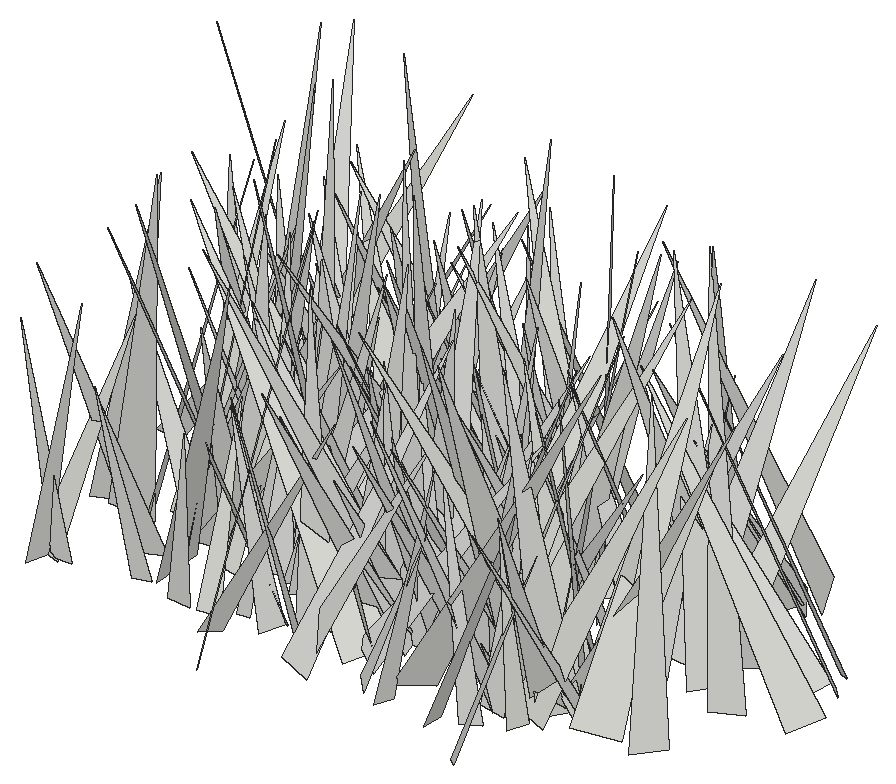
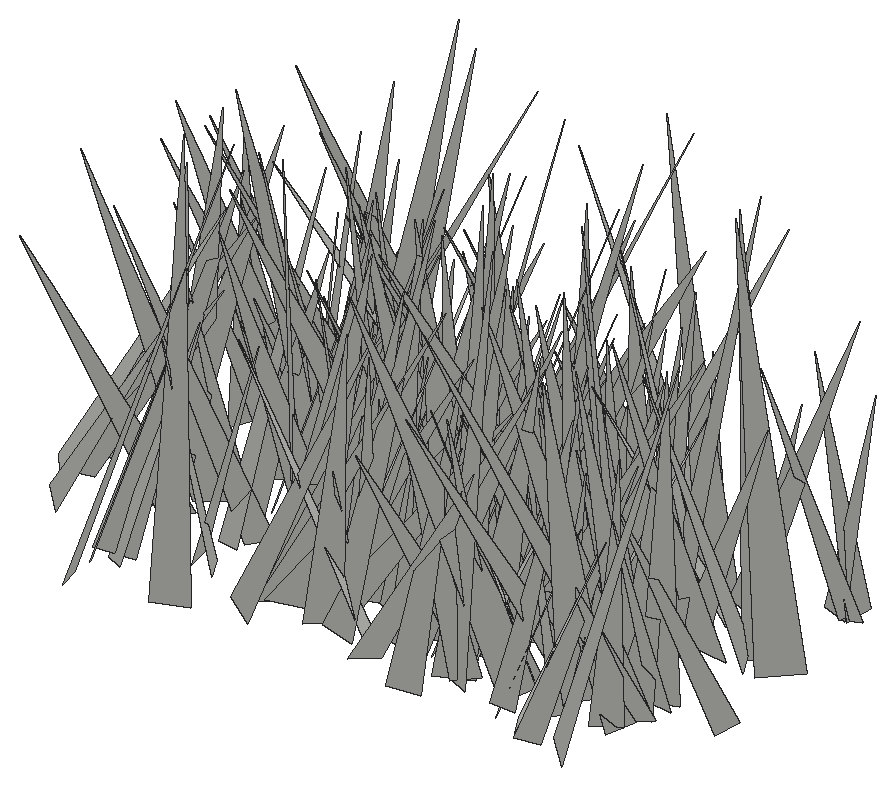
# SketchUp Ruby script. Lengths in inches.
U = 1.inch
M = Sketchup.active_model
def pt(a) = Geom::Point3d.new(a.map { |v| v * U })
def face(e, loops, mat)
  f = e.add_face(loops[0].map { |a| pt(a) })
  loops[1..].each { |l| e.add_face(l.map { |a| pt(a) }).erase! }
  f.material = f.back_material = mat if mat
  f
end
# faces: each face lists its corners as indices into pts; further lists are holes
def faces(e, pts, list, mat = nil) = list.each { |f| face(e, (f[0].is_a?(Array) ? f : [f]).map { |l| l.map { |i| pts[i] } }, mat) }
# xy, xz, yz: faces in a plane at the given z, y or x. An outline is a flat list of corners, or four numbers for a rectangle; further outlines are holes
def ring(l) = l.size == 4 ? [[l[0], l[1]], [l[2], l[1]], [l[2], l[3]], [l[0], l[3]]] : l.each_slice(2).to_a
def flat(e, list, mat, &to3) = list.each { |f| face(e, (f[0].is_a?(Array) ? f : [f]).map { |l| ring(l).map { |u, v| to3.(u, v) } }, mat) }
def xy(e, z, list, mat = nil) = flat(e, list, mat) { |x, y| [x, y, z] }
def xz(e, y, list, mat = nil) = flat(e, list, mat) { |x, z| [x, y, z] }
def yz(e, x, list, mat = nil) = flat(e, list, mat) { |y, z| [x, y, z] }
def lines(e, pts, list) = list.each { |a, b| e.add_line(pt(pts[a]), pt(pts[b])) }
# prism: a flat outline (further loops are holes) pulled along v
def prism(e, loops, v, mat = nil)
  f = face(e, loops, mat); d = Geom::Vector3d.new(v.map { |x| x * U })
  f.pushpull(f.normal.samedirection?(d) ? d.length : -d.length)
end
def box(e, o, s, mat = nil) = prism(e, [[o, [o[0] + s[0], o[1], o[2]], [o[0] + s[0], o[1] + s[1], o[2]], [o[0], o[1] + s[1], o[2]]]], [0, 0, s[2]], mat)
def at(x, y, z, deg = 0) = Geom::Transformation.translation(pt([x, y, z])) * Geom::Transformation.rotation(ORIGIN, Z_AXIS, deg.degrees)
def axes(o, x, y, z) = Geom::Transformation.new([*x, 0, *y, 0, *z, 0, *pt(o).to_a, 1])
def part(name) = M.definitions.add(name)
# library, detail: a bought-in or finely detailed component or shape, given as its bounding box
def library(name, o, s) = part(name).tap { |d| box(d.entities, o, s) }
def detail(e, o, s) = box(e.add_group.entities, o, s)
def put(e, d, t, mat = nil) = e.add_instance(d, t).tap { |i| i.material = mat if mat }
def group(e, t, mat = nil) = e.add_group.tap { |g| g.transformation = t; g.material = mat if mat }.entities
root = M.entities
c1 = part("fur_instance\#9")
p = [[0.8125,0,1.79],[0.67,-0.02,1.48],[0,-0.11,0],[0,0.11,0]]
faces(c1.entities,p,[[0,1,2,3]])
put(root,c1,axes([508.12,72.6,-21.86],[0.58274,-3.68979,0.92218],[-3.78198,-0.46356,0.53511],[0.40205,0.98748,3.697]))
put(root,c1,axes([511.35,69.62,-21.66],[6.37842,4.90538,1.53696],[4.59516,-6.53882,1.79932],[-2.30422,0.53885,7.84279]))
put(root,c1,axes([516.26,72.1,-21.86],[2.61371,2.45973,0.53308],[2.49517,-2.43181,-1.01309],[0.32949,-1.09634,3.44317]))
put(root,c1,axes([512.71,73.15,-21.86],[-3.88391,-3.01754,1.00768],[-2.99103,4.00531,0.46572],[1.08383,0.24005,4.89626]))
put(root,c1,axes([506.625,74.36,-21.86],[8.18505,-1.50624,0.16494],[-1.43272,-7.98824,-1.85106],[-0.49323,-1.79175,8.11402]))
put(root,c1,axes([517.57,71.6,-21.86],[4.20313,-0.16718,1.34956],[-0.39887,-4.34286,0.70427],[-1.30006,0.79192,4.14708]))
put(root,c1,axes([503.32,72.43,-21.86],[-0.94166,-4.10224,1.61468],[-4.38512,0.70145,-0.77524],[-0.45421,1.73259,4.13692]))
put(root,c1,axes([502.62,72.03,-21.86],[4.80103,-0.44543,1.50068],[-0.59366,-4.99749,0.41591],[-1.44845,0.57184,4.80368]))
put(root,c1,axes([520.4375,73.95,-21.86],[-5.1626,-2.88411,0.4563],[-2.82641,5.16852,0.6903],[0.7333,-0.3834,5.87316]))
put(root,c1,axes([513.81,71.89,-21.66],[2.98745,4.37857,0.43851],[4.21633,-2.69647,-1.80015],[1.25963,-1.35874,4.98559]))
put(root,c1,axes([522.24,74.51,-21.86],[2.51881,-4.55482,0.15905],[-4.51842,-2.51942,-0.59372],[-0.59628,-0.14918,5.17091]))
put(root,c1,axes([510.13,71.75,-21.86],[4.70172,-1.10111,0.26171],[-1.12934,-4.49092,1.39405],[0.07438,1.41645,4.62334]))
put(root,c1,axes([506.19,73.04,-21.86],[-0.09942,-3.58739,1.13729],[-3.70553,-0.10534,-0.65623],[-0.65715,1.13676,3.52826]))
put(root,c1,axes([523.46,74.95,-21.86],[-3.70308,-3.24105,0.05421],[-3.08159,3.54543,1.46762],[1.00557,-1.07036,4.69716]))
put(root,c1,axes([520.76,72.2,-21.86],[-0.54656,4.2534,1.19948],[4.32093,0.26075,1.04426],[-0.92722,-1.29209,4.15928]))
put(root,c1,axes([515.43,75,-21.66],[1.43774,-5.64122,0.58152],[-5.34924,-1.54822,-1.79367],[-1.88339,0.09091,5.53834]))
put(root,c1,axes([522.07,73.05,-21.86],[-3.10303,1.40825,1.48641],[1.65077,3.31728,0.3033],[1.21143,-0.91317,3.39411]))
put(root,c1,axes([511.62,73.125,-21.86],[-3.58724,1.8714,1.40372],[2.1412,3.66165,0.59026],[0.94225,-1.19623,4.00275]))
put(root,c1,axes([520.34,76.11,-21.86],[6.29678,-5.28708,1.00032],[-4.88133,-6.26054,-2.36253],[-2.26416,-1.20654,7.87535]))
put(root,c1,axes([511.5,73.86,-21.86],[-4.9129,-5.75828,0.52895],[-5.68371,4.68095,-1.83254],[-1.06438,1.58274,7.34412]))
put(root,c1,axes([515.98,75.3,-21.66],[-8.04638,-2.10125,0.20494],[-2.02323,7.90531,1.61682],[0.60315,-1.51404,8.15753]))
put(root,c1,axes([517.01,75.45,-21.66],[-6.19203,-3.31038,1.54754],[-2.85802,6.28451,2.00782],[2.2771,-1.114,6.72819]))
put(root,c1,axes([505.65,74.35,-21.66],[-0.4063,-5.76079,1.26429],[-5.69006,0.04941,-1.60344],[-1.5519,1.32705,5.54804]))
put(root,c1,axes([502.58,72.48,-21.86],[0.61438,4.77457,1.24038],[4.786,-0.27399,-1.3159],[1.1955,-1.35681,4.63059]))
put(root,c1,axes([523.04,75.625,-21.86],[-8.10416,-1.22815,0.06312],[-1.16757,7.81624,2.17553],[0.38615,-2.14192,7.90272]))
put(root,c1,axes([519.85,71.31,-21.66],[6.47636,2.00005,0.90058],[1.74291,-6.39683,1.67254],[-1.33173,1.35459,6.56857]))
put(root,c1,axes([517.88,72.83,-21.66],[7.15691,-3.14413,0.26361],[-3.09126,-6.8566,2.14652],[0.63178,2.06831,7.5166]))
put(root,c1,axes([519.76,76.26,-21.86],[0.59961,-8.00132,0.48644],[-8.01433,-0.60861,-0.13198],[-0.1682,0.47514,8.02267]))
put(root,c1,axes([518.91,75.29,-21.86],[0.11807,-5.18176,0.38422],[-4.95689,-0.22756,-1.54584],[-1.55804,0.33133,4.94722]))
put(root,c1,axes([509.3,72.66,-21.86],[-0.85461,3.70026,0.75554],[3.7566,0.91253,-0.21994],[0.38824,-0.68446,3.79129]))
put(root,c1,axes([522.61,74.59,-21.86],[4.49335,-4.83843,2.48866],[-4.8443,-5.0271,-1.02712],[-2.47721,1.05444,6.5227]))
put(root,c1,axes([513.84,71.52,-21.86],[1.69788,6.23349,0.03172],[6.16311,-1.67374,-0.97718],[0.93461,-0.28707,6.38626]))
put(root,c1,axes([520.75,73.36,-21.86],[0.78552,4.64999,1.51438],[4.88897,-0.70993,-0.35606],[0.11721,-1.55126,4.70241]))
put(root,c1,axes([519.375,76.59,-21.86],[-4.17954,-4.03403,0.06779],[-3.83281,4.00041,1.74723],[1.26,-1.21235,5.53978]))
put(root,c1,axes([521.85,69.87,-21.86],[5.70548,5.18554,0.14342],[4.71826,-5.27598,3.06024],[-2.15603,2.1765,7.07653]))
put(root,c1,axes([512.72,74.08,-21.86],[-1.61639,5.70202,2.80279],[6.31476,1.76115,0.05886],[0.70173,-2.71416,5.92641]))
put(root,c1,axes([515.04,76.29,-21.66],[3.98276,-1.20965,1.22676],[-0.42908,-3.68899,-2.24451],[-1.66855,-1.93873,3.5054]))
put(root,c1,axes([514.28,75.85,-21.86],[-4.07436,-2.22938,0.28557],[-2.14023,4.02883,0.91657],[0.68639,-0.67121,4.55307]))
put(root,c1,axes([514.71,74.17,-21.66],[-5.12266,-6.1706,2.10185],[-6.50165,4.64284,-2.21548],[-0.47189,3.01719,7.70776]))
put(root,c1,axes([515.17,73.78,-21.86],[-5.23637,6.32875,0.17784],[5.87309,4.76933,3.20385],[-2.36465,-2.16904,7.5636]))
put(root,c1,axes([515.23,73.57,-21.86],[2.725,5.40327,0.30402],[4.86473,-2.29653,-2.78814],[2.3711,-1.498,5.37096]))
put(root,c1,axes([518.57,75.48,-21.86],[-1.2496,-4.95098,2.04852],[-4.91628,1.89585,1.58307],[2.13046,1.47094,4.85465]))
put(root,c1,axes([507.4,76.77,-21.86],[4.3108,-3.69492,0.61953],[-3.55093,-4.33068,-1.12044],[-1.19463,-0.46051,5.56597]))
put(root,c1,axes([521.83,73.84,-21.86],[0.86928,6.52033,1.58307],[6.24969,-0.2059,-2.58369],[2.44176,-1.79425,6.04937]))
put(root,c1,axes([503.125,76.37,-21.86],[1.84601,-7.44066,1.73932],[-7.59322,-1.58595,1.27441],[0.85535,1.97933,7.55956]))
put(root,c1,axes([515.2,76.85,-21.86],[2.62732,-3.98087,0.28129],[-3.95197,-2.64215,-0.47983],[-0.55532,-0.03119,4.74551]))
put(root,c1,axes([510.52,72.98,-21.66],[2.07794,4.44656,0.23399],[4.16362,-2.03187,1.63715],[-1.57826,0.49406,4.62704]))
put(root,c1,axes([526.51,74.42,-21.86],[-5.32179,3.05618,1.70346],[3.04909,5.5718,-0.47069],[1.71611,-0.42222,6.11884]))
put(root,c1,axes([502.13,76.76,-21.86],[4.60789,-6.31495,1.14074],[-6.41656,-4.51508,0.92427],[0.08686,1.46561,7.76253]))
put(root,c1,axes([505.51,78.7,-21.86],[-3.16063,-7.46069,0.64697],[-7.21635,3.22195,1.90087],[2.00118,-0.16476,7.87643]))
put(root,c1,axes([515.02,75.65,-21.86],[-0.34045,4.62028,2.07312],[5.05885,0.21591,0.34957],[-0.23002,-2.08976,4.6196]))
put(root,c1,axes([516.96,74.91,-21.86],[3.82826,-1.89723,1.31218],[-2.241,-3.66166,1.2438],[-0.54703,1.72325,4.08754]))
put(root,c1,axes([505.73,76.51,-21.86],[3.31192,-3.28223,0.0309],[-3.2384,-3.26025,0.79144],[0.53549,0.5836,4.59516]))
put(root,c1,axes([513.31,76.02,-21.86],[5.02607,-4.57327,2.19343],[-4.92834,-5.13329,0.59007],[-1.19892,1.92923,6.76964]))
put(root,c1,axes([523.01,75.75,-21.86],[1.98838,-4.24744,1.75797],[-4.57109,-1.62434,1.24561],[0.4862,2.09896,4.52138]))
put(root,c1,axes([520.94,78.43,-21.86],[-3.46675,-5.54657,1.13696],[-5.08588,3.63649,2.23277],[2.48816,-0.29493,6.14797]))
put(root,c1,axes([522.9,75.58,-21.86],[-4.62696,-2.40171,1.71965],[-2.7299,4.69747,-0.78458],[1.12828,1.51649,5.15378]))
put(root,c1,axes([514.03,76.47,-21.86],[-4.61226,3.61546,0.79034],[3.61757,4.1381,2.18138],[-0.78062,-2.18488,5.43931]))
put(root,c1,axes([519,74.41,-21.86],[-5.68198,1.58826,2.45655],[1.00817,6.10119,-1.61279],[2.74605,1.04639,5.67506]))
put(root,c1,axes([519.86,79.15,-21.86],[-5.63617,-2.55407,1.20627],[-1.85262,5.37498,2.72438],[2.13217,-2.08115,5.55585]))
put(root,c1,axes([522.65,75.18,-21.86],[6.21247,-1.9108,0.54363],[-1.98453,-5.88708,1.9863],[0.09123,2.05733,6.18874]))
put(root,c1,axes([506.47,76.24,-21.86],[3.95823,-3.37287,0.12226],[-3.1364,-3.60629,2.0534],[1.24667,1.63622,4.7778]))
put(root,c1,axes([517.1875,77.24,-21.66],[-2.08811,-4.65792,0.59921],[-4.45757,1.75934,-1.85749],[-1.47829,1.27435,4.7546]))
put(root,c1,axes([521.63,76.63,-21.86],[-4.54367,3.48057,1.82928],[3.81076,4.58683,0.73803],[0.96889,-1.71821,5.67579]))
put(root,c1,axes([506.05,76.54,-21.86],[-3.48001,3.233,0.8636],[3.33945,3.27515,1.19585],[-0.21495,-1.45934,4.59703]))
put(root,c1,axes([516.31,74.93,-21.66],[1.43872,7.93621,2.15807],[7.82752,-1.99366,2.11323],[-2.52399,-1.65906,7.7838]))
put(root,c1,axes([509.97,76.45,-21.86],[2.74788,4.31889,0.7575],[4.17328,-2.30167,-2.01583],[1.34551,-1.68135,4.70533]))
put(root,c1,axes([508.06,75.3,-21.86],[0.74131,3.87524,0.12897],[3.87698,-0.74271,0.03187],[-0.05555,-0.12068,3.94537]))
put(root,c1,axes([507.4375,77.28,-21.86],[-4.12278,4.06528,3.37823],[4.64279,4.83304,-0.14992],[2.52655,-2.24755,5.78803]))
put(root,c1,axes([512.39,78.32,-21.86],[-0.32554,-5.06602,0.7464],[-4.99056,0.14633,-1.18345],[-1.14716,0.80105,4.9366]))
put(root,c1,axes([524.4,74.24,-21.86],[-3.86216,7.0455,1.20437],[6.7899,4.04407,-1.88376],[2.2331,-0.11104,7.81068]))
put(root,c1,axes([515.91,76.46,-21.86],[-0.78367,4.54033,1.31363],[4.69244,0.5877,0.76808],[-0.56674,-1.41222,4.54299]))
put(root,c1,axes([506.01,75.78,-21.86],[6.26441,4.08516,1.86388],[4.05019,-6.52197,0.68206],[-1.9387,-0.42509,7.44756]))
put(root,c1,axes([509.68,77.84,-21.86],[-4.95355,2.49117,1.9463],[2.93301,4.97148,1.10159],[1.17959,-1.90003,5.43416]))
put(root,c1,axes([522.27,78.33,-21.86],[-3.91317,-2.34388,0.53173],[-2.28614,3.94348,0.55853],[0.74167,-0.21123,4.52711]))
put(root,c1,axes([518.65,75.03,-21.66],[2.72489,7.5123,0.23605],[7.26372,-2.56761,-2.13568],[1.931,-0.94238,7.70056]))
put(root,c1,axes([509.48,76.12,-21.86],[-0.20928,5.81187,1.2771],[5.90875,0.05179,0.73257],[-0.70395,-1.2931,5.76932]))
put(root,c1,axes([510.41,76.12,-21.86],[5.34451,-1.51745,2.02584],[-2.07356,-5.33917,1.4711],[-1.45157,2.03988,5.35746]))
put(root,c1,axes([523.12,76.59,-21.86],[0.51844,5.23573,1.343],[5.13497,-0.0558,-1.76472],[1.68777,-1.43851,4.95655]))
put(root,c1,axes([512.31,78.95,-21.86],[0.02895,-4.95019,0.58964],[-4.94989,0.0415,0.59139],[0.59214,0.58889,4.91483]))
put(root,c1,axes([518.45,76.64,-21.86],[-4.21104,-1.2398,0.43934],[-1.31531,3.95873,-1.43574],[-0.00925,1.50143,4.14832]))
put(root,c1,axes([517.09,77.91,-21.86],[3.85978,2.30102,0.3483],[2.28006,-3.60384,-1.45862],[0.46617,-1.42533,4.2503]))
put(root,c1,axes([509.1,77.8,-21.86],[-4.69197,-2.31538,0.05263],[-2.28134,4.60011,-1.00642],[-0.39908,0.92541,5.13447]))
put(root,c1,axes([506.0625,74.81,-21.66],[4.52328,4.39752,0.22155],[4.10164,-4.32376,2.0806],[-1.60118,1.34692,5.95561]))
put(root,c1,axes([513.91,78.67,-21.86],[3.13383,-5.16211,1.39491],[-5.34355,-3.08346,0.59403],[-0.19921,1.50298,6.00961]))
put(root,c1,axes([510.9375,75.66,-21.86],[-6.51752,1.2418,2.00991],[0.54856,6.53189,-2.25684],[2.29801,1.9627,6.23913]))
put(root,c1,axes([511.25,78.33,-21.86],[-3.24563,2.42896,0.17461],[2.25293,2.88449,1.75171],[-0.92447,-1.49811,3.65588]))
put(root,c1,axes([514.92,80.65,-21.86],[-0.43608,-7.58063,0.50958],[-7.59761,0.43802,0.01424],[0.04352,0.50791,7.59315]))
put(root,c1,axes([510.28,77.16,-21.86],[-3.93894,0.78438,0.2139],[0.7314,3.88076,-0.76228],[0.35506,0.70765,3.94328]))
put(root,c1,axes([515.53,78.02,-21.86],[-4.0044,1.49429,0.5536],[1.5481,4.00291,0.3933],[0.37782,-0.56428,4.25599]))
put(root,c1,axes([514.53,78.76,-21.86],[-1.30736,-3.53096,1.01989],[-3.67333,1.2908,-0.2398],[0.12042,1.04076,3.75757]))
put(root,c1,axes([513.12,80.63,-21.86],[-3.83453,-4.44323,0.31037],[-4.29048,3.7947,1.3169],[1.19597,-0.63261,5.71941]))
put(root,c1,axes([518.69,78.18,-21.86],[3.7348,-2.45498,0.02516],[-2.33086,-3.53122,1.44009],[0.77113,1.21649,4.23106]))
put(root,c1,axes([509.13,77.04,-21.86],[2.12896,3.50938,0.78952],[3.35263,-2.26833,1.04217],[-1.30344,-0.10245,3.97015]))
put(root,c1,axes([520.75,76.76,-21.66],[6.22186,3.72093,2.03459],[3.43335,-6.54009,1.46143],[-2.48938,0.27987,7.10078]))
put(root,c1,axes([519.51,78.05,-21.86],[7.2049,-3.47591,1.96261],[-3.83046,-7.15988,1.38131],[-1.1231,2.12096,7.87937]))
put(root,c1,axes([511.93,82.83,-21.86],[-6.50454,-4.83681,0.42708],[-4.2184,5.98256,3.50717],[2.40464,-2.5885,7.30777]))
put(root,c1,axes([503.68,76.625,-21.86],[5.51365,3.20537,1.24598],[2.89904,-5.59864,1.57419],[-1.84998,0.77981,6.18035]))
put(root,c1,axes([521.63,81.5625,-21.66],[-2.90473,-5.90083,0.221],[-5.68544,2.86131,1.67173],[1.5951,-0.54696,6.36102]))
put(root,c1,axes([514.91,77.8,-21.66],[2.90433,5.023,0.38727],[4.82562,-2.64532,-1.87916],[1.44702,-1.25991,5.48948]))
put(root,c1,axes([522.5625,79.43,-21.86],[-4.35819,2.96505,1.59627],[3.3258,4.19926,1.28011],[0.52792,-1.97688,5.11338]))
put(root,c1,axes([525.29,80.72,-21.86],[1.43067,-7.01564,1.7352],[-6.90944,-1.84641,-1.76845],[-2.11892,1.28394,6.9382]))
put(root,c1,axes([529.43,79.04,-21.86],[-4.14935,5.21761,0.66717],[4.85978,3.47746,3.02911],[-2.01273,-2.35998,5.93844]))
put(root,c1,axes([512.66,82.05,-21.86],[5.40488,-4.57462,0.50738],[-4.27322,-5.27816,-2.06831],[-1.71004,-1.26929,6.77215]))
put(root,c1,axes([514.7,77.93,-21.86],[-3.77046,5.93467,2.17976],[6.06315,4.1134,-0.71146],[1.79161,-1.43096,6.99504]))
put(root,c1,axes([518.43,79.07,-21.86],[0.00091,-3.67707,1.93886],[-4.08733,0.35251,0.67045],[0.75747,1.90654,3.61543]))
put(root,c1,axes([504.85,77.16,-21.86],[0.72086,7.11073,0.81641],[7.15729,-0.71063,-0.13028],[0.04812,-0.82534,7.14599]))
put(root,c1,axes([508.7,78.96,-21.66],[-2.86629,5.19134,1.30889],[5.27356,2.48156,1.70596],[-0.92348,-1.94182,5.67938]))
put(root,c1,axes([509.05,77.47,-21.66],[-0.59602,7.49567,1.64856],[6.68012,1.32078,-3.59019],[3.77872,-1.15261,6.60687]))
put(root,c1,axes([525.4375,79.125,-21.86],[-5.88987,4.84378,2.23578],[5.14185,6.04195,0.45575],[1.42207,-1.78441,7.61217]))
put(root,c1,axes([523.4,78.66,-21.86],[0.22863,4.55848,1.01522],[4.65358,-0.13679,-0.43379],[0.39321,-1.03161,4.54355]))
put(root,c1,axes([504.91,80.97,-21.66],[1.45023,-6.39796,1.08768],[-6.25164,-1.07813,1.99368],[1.74182,1.45734,6.24998]))
put(root,c1,axes([504.21,82.1,-21.86],[2.77965,-6.05851,0.20454],[-6.05263,-2.78627,-0.276],[-0.3362,0.0706,6.66001]))
put(root,c1,axes([510.05,80.24,-21.86],[-6.653,2.83628,0.09553],[2.75112,6.38619,1.99099],[-0.69638,-1.86767,6.95291]))
put(root,c1,axes([512.22,80.92,-21.86],[-0.4517,-7.27096,2.0225],[-7.50286,0.65147,0.6664],[0.81515,1.96726,7.25444]))
put(root,c1,axes([508.56,79.94,-21.86],[6.38697,-1.69717,1.73981],[-1.81592,-6.58358,0.24416],[-1.61547,0.69051,6.6041]))
put(root,c1,axes([517.57,76.93,-21.86],[-1.37451,8.097,0.63904],[7.82187,1.49419,-2.10823],[2.18815,-0.25501,7.93763]))
put(root,c1,axes([518.75,78.4375,-21.86],[3.29752,4.92899,1.52703],[4.76096,-3.60504,1.35547],[-1.98997,-0.45731,5.77332]))
put(root,c1,axes([505.89,80.25,-21.86],[4.80804,6.17674,2.98381],[6.78482,-4.81897,-0.95722],[-1.01068,-2.96612,7.76873]))
put(root,c1,axes([526.88,78.07,-21.86],[-0.02832,7.80203,1.3013],[7.5934,-0.33756,2.1891],[-2.2148,-1.25708,7.48868]))
put(root,c1,axes([509.68,78.04,-21.86],[-7.86516,0.65945,1.92725],[0.13584,7.83978,-2.12819],[2.03241,2.02799,7.60042]))
put(root,c1,axes([508.59,80.11,-21.86],[3.89931,-1.45547,0.98195],[-1.58431,-3.9476,0.44006],[-0.75669,0.76505,4.13877]))
put(root,c1,axes([528.46,80.85,-21.66],[-4.24155,2.82864,0.08548],[2.61337,3.85608,2.07369],[-1.08573,-1.76881,4.65744]))
put(root,c1,axes([504.07,80.75,-21.86],[2.29625,-5.32789,2.30917],[-5.72704,-2.48806,-0.04565],[-0.95905,2.10109,5.80148]))
put(root,c1,axes([515.39,81.09,-21.86],[3.99451,-5.40043,2.70776],[-5.64329,-4.49426,-0.63847],[-2.15638,1.75774,6.68679]))
put(root,c1,axes([515.27,81.3,-21.86],[-1.72033,-4.15588,1.09836],[-4.2769,1.77348,0.01157],[0.4311,1.01028,4.49785]))
put(root,c1,axes([508.74,79.99,-21.86],[0.17252,3.92598,1.26935],[3.97591,-0.49782,0.99933],[-1.10305,-1.18034,3.80058]))
put(root,c1,axes([517.62,81.25,-21.86],[-2.41735,-5.08882,0.8159],[-4.81582,1.90935,-2.35956],[-1.83565,1.69223,5.11586]))
put(root,c1,axes([509.97,81.28,-21.86],[-5.02237,2.51021,1.68016],[2.86774,4.98644,1.12241],[0.94877,-1.78398,5.50142]))
put(root,c1,axes([504.375,81.58,-21.66],[1.31964,-4.20384,0.49444],[-3.9297,-1.02429,1.77946],[1.57296,0.96785,4.03079]))
put(root,c1,axes([501.02,80.96,-21.66],[2.58418,-3.37784,0.00054],[-2.92311,-2.23595,2.1316],[1.69269,1.29557,3.68023]))
put(root,c1,axes([518,79.82,-21.86],[-6.07575,2.79462,0.62219],[2.80321,6.10345,-0.04049],[0.58225,-0.22305,6.68752]))
put(root,c1,axes([529.08,81.14,-21.66],[-5.24888,-4.54366,0.15791],[-4.36596,4.97023,-2.11085],[-1.26815,1.69482,6.61361]))
put(root,c1,axes([515.91,79.99,-21.86],[3.41828,7.22194,2.57308],[7.56489,-3.63472,0.1519],[-1.24484,-2.25703,7.98861]))
put(root,c1,axes([507.99,80.13,-21.86],[-2.49427,4.27012,1.59064],[4.35584,2.76683,-0.59729],[1.33819,-1.04698,4.90903]))
put(root,c1,axes([510.9,79.18,-21.86],[-2.09774,5.99421,0.07606],[5.73274,1.98235,1.88224],[-1.75272,-0.69034,6.06533]))
put(root,c1,axes([508.17,79.82,-21.86],[4.9565,-0.0282,0.53243],[-0.1703,-4.80111,1.33099],[-0.50525,1.34155,4.77453]))
put(root,c1,axes([516.57,82.39,-21.86],[-3.87512,-3.17972,0.32504],[-3.163,3.88842,0.32938],[0.4601,-0.04943,5.00187]))
put(root,c1,axes([524.2,84.34,-21.66],[4.00993,-5.51552,0.33203],[-5.14979,-3.87921,-2.24547],[-2.00271,-1.06842,6.43882]))
put(root,c1,axes([513.36,82.78,-21.86],[-2.38013,-2.88459,0.25848],[-2.75196,2.35686,0.96161],[0.90246,-0.42079,3.61403]))
put(root,c1,axes([523.85,79.53,-21.66],[-1.22058,7.14872,1.6543],[7.02907,1.62036,-1.81584],[2.10547,-1.26529,7.02116]))
put(root,c1,axes([518.5,83.2,-21.66],[-6.87561,-0.89332,0.66489],[-0.69538,6.69239,1.80069],[0.86979,-1.71115,6.69549]))
put(root,c1,axes([517.86,83.2,-21.86],[3.87648,-5.20572,1.47803],[-5.00062,-4.14086,-1.46909],[-2.0683,0.2548,6.32205]))
put(root,c1,axes([519.4375,80.69,-21.86],[6.18055,4.14964,3.19418],[4.26505,-6.85588,0.65402],[-3.03836,-1.18276,7.41558]))
put(root,c1,axes([520.92,80.75,-21.66],[0.63179,6.0642,2.01169],[5.81387,0.29266,-2.70812],[2.6496,-2.08816,5.46258]))
put(root,c1,axes([517.0625,82.23,-21.86],[-0.19276,-5.01478,1.27598],[-5.16585,0.1124,-0.33865],[-0.30027,1.28555,5.00705]))
put(root,c1,axes([516.1,82.18,-21.66],[-2.43401,-4.94438,0.27236],[-4.40728,2.02468,-2.63096],[-2.25763,1.37813,4.84245]))
put(root,c1,axes([510.44,83.65,-21.86],[4.15376,-5.21591,0.7578],[-5.12927,-4.22232,-0.94677],[-1.21268,-0.00681,6.60024]))
put(root,c1,axes([518.28,80.34,-21.86],[6.10707,-2.19869,2.10682],[-2.76305,-5.98564,1.76265],[-1.28003,2.43046,6.24689]))
put(root,c1,axes([515.27,83.73,-21.86],[-2.01035,-7.12989,1.00319],[-7.18316,2.0575,0.22838],[0.49393,0.90254,7.40437]))
put(root,c1,axes([518.43,83.36,-21.86],[-6.42762,0.7775,0.36666],[0.8533,6.10569,2.01137],[0.10407,-2.04186,6.15412]))
put(root,c1,axes([512.45,83.61,-21.66],[-0.7364,-6.55979,0.93298],[-6.36781,0.44127,-1.92351],[-1.83094,1.10364,6.31453]))
put(root,c1,axes([511.02,81.09,-21.86],[-4.49285,4.90641,0.97236],[5.00159,4.41981,0.80831],[0.04935,-1.26349,6.60342]))
put(root,c1,axes([503.89,80.92,-21.86],[0.3484,4.1984,0.59349],[4.23915,-0.35779,0.04247],[-0.09183,-0.58788,4.21262]))
put(root,c1,axes([518.64,81.19,-21.86],[-5.45873,5.352,1.02249],[5.44819,5.38274,0.9113],[0.08123,-1.36725,7.5902]))
put(root,c1,axes([516.89,80.28,-21.66],[-6.05954,0.33778,0.89505],[0.02694,5.79744,-2.00555],[0.95629,1.97708,5.728]))
put(root,c1,axes([528.34,82.44,-21.86],[-3.48224,-3.77241,0.29956],[-3.58403,3.15695,-1.90663],[-1.21472,1.49981,4.76674]))
put(root,c1,axes([508.51,82.29,-21.86],[3.59656,-0.31618,0.04156],[-0.31764,-3.59357,0.14939],[-0.02828,0.15246,3.60734]))
put(root,c1,axes([524.49,85.28,-21.66],[-4.06772,-3.26977,0.32403],[-2.78571,3.7053,2.41936],[1.74246,-1.70943,4.62433]))
put(root,c1,axes([510.36,83.01,-21.86],[-3.2308,-2.41105,0.08917],[-2.40238,3.20101,-0.49122],[-0.22293,0.4467,4.00124]))
put(root,c1,axes([506.2,83.48,-21.86],[3.91302,0.34843,0.25725],[0.41449,-3.69091,-1.30566],[-0.12562,-1.32482,3.70519]))
put(root,c1,axes([503.96,82.51,-21.86],[6.68383,-3.60485,0.36068],[-3.59385,-6.50181,1.61538],[0.45749,1.59067,7.42019]))
put(root,c1,axes([522.08,82.53,-21.86],[-4.57594,-0.69447,0.70937],[-0.73517,4.61906,-0.2203],[0.6671,0.32667,4.62309]))
put(root,c1,axes([508,82.27,-21.86],[4.04604,3.23344,0.3968],[3.2461,-3.94826,-0.92578],[0.27467,-0.96906,5.09593]))
put(root,c1,axes([507.96,84.18,-21.86],[0.4513,-4.46287,0.47479],[-4.46772,-0.49211,-0.3789],[-0.42669,0.43236,4.4696]))
put(root,c1,axes([524.08,84.52,-21.86],[-2.1706,-3.79382,0.07549],[-3.76138,2.16267,0.53397],[0.50075,-0.20018,4.33814]))
put(root,c1,axes([505.9,83.34,-21.86],[2.36967,1.89121,2.13493],[2.35412,-2.86396,-0.07595],[-1.61018,-1.40392,3.03088]))
put(root,c1,axes([516.75,81.14,-21.86],[0.6459,3.9486,0.07217],[3.68247,-0.62859,1.43463],[-1.42692,0.16515,3.73504]))
put(root,c1,axes([504.46,83.05,-21.86],[2.60909,-3.89298,2.22887],[-4.24925,-2.97119,-0.21539],[-1.4377,1.71676,4.68148]))
put(root,c1,axes([524.46,80.69,-21.86],[-1.13308,6.40977,0.66119],[6.08836,1.28481,-2.02171],[2.11049,-0.26515,6.18722]))
put(root,c1,axes([505.9,85.43,-21.86],[3.91388,-2.85851,1.41513],[-2.09693,-3.9939,-2.26798],[-2.40345,-1.17037,4.2832]))
put(root,c1,axes([510.09,82.04,-21.86],[0.83118,5.18677,1.07004],[5.28228,-0.88982,0.21009],[-0.38088,-1.02179,5.24874]))
put(root,c1,axes([504.96,81.04,-21.66],[-7.30658,0.78889,2.52937],[0.00726,7.42557,-2.29501],[2.64953,2.15518,6.98151]))
put(root,c1,axes([521.2,82.83,-21.86],[-3.23487,-1.73884,2.61208],[-2.22596,3.91581,-0.14997],[2.2117,1.39779,3.66954]))
put(root,c1,axes([510.52,83.7,-21.86],[-2.90002,-7.26429,3.03178],[-7.85451,2.88308,-0.60516],[0.51793,3.0479,7.79832]))
put(root,c1,axes([507.98,83.03,-21.86],[5.9864,-4.39629,0.74457],[-4.35138,-5.48795,2.58196],[0.97326,2.50473,6.96403]))
put(root,c1,axes([513.34,84.7,-21.66],[-6.69596,1.51903,0.23584],[1.52209,6.40398,1.96756],[-0.2152,-1.96993,6.57815]))
put(root,c1,axes([524.53,86.33,-21.86],[-7.22673,-3.69522,1.05519],[-3.3656,7.17065,2.06111],[1.85494,-1.38592,7.85061]))
put(root,c1,axes([506.77,81.72,-21.66],[5.85572,0.96623,0.0245],[0.91904,-5.61274,1.69591],[-0.29926,1.66948,5.68743]))
put(root,c1,axes([509.88,83.71,-21.66],[-0.77614,4.62516,2.62163],[4.88719,1.66369,-1.48826],[2.09294,-2.16967,4.44742]))
put(root,c1,axes([520.625,85.91,-21.66],[0.39282,-7.92697,1.06347],[-7.86049,-0.18606,1.51663],[1.47665,1.11832,7.79044]))
put(root,c1,axes([514.55,83.08,-21.86],[4.96423,2.67259,0.04648],[2.6631,-4.93667,-0.5706],[0.22978,-0.52435,5.60898]))
put(root,c1,axes([511.2,85.35,-21.86],[1.67149,-5.33301,0.8085],[-5.34441,-1.75188,-0.5067],[-0.72935,0.6152,5.5658]))
put(root,c1,axes([507.88,84.46,-21.86],[-3.47734,-1.80435,0.22841],[-1.8088,3.48242,-0.02761],[0.19,0.12974,3.9175]))
put(root,c1,axes([518.59,84.76,-21.66],[-2.94744,-5.34651,0.76174],[-5.29498,2.69026,-1.60576],[-1.06233,1.42484,5.89017]))
put(root,c1,axes([516.11,83.44,-21.86],[-4.47005,3.93119,1.60818],[4.11701,4.5843,0.23722],[1.04438,-1.24571,5.94805]))
put(root,c1,axes([503.67,82.31,-21.66],[1.59933,7.72158,1.03232],[7.26868,-1.09996,-3.03359],[2.80263,-1.55359,7.2786]))
put(root,c1,axes([510.63,82.33,-21.66],[-3.36626,3.2291,1.55087],[2.48228,3.63709,-2.18492],[2.58275,0.71309,4.12128]))
put(root,c1,axes([504.65,85.38,-21.86],[-5.20648,-5.71637,1.32602],[-5.85189,5.18966,-0.6046],[0.43665,1.3904,7.70836]))
put(root,c1,axes([506.85,84.78,-21.86],[-3.58425,-2.16039,0.18109],[-2.16614,3.55434,-0.47063],[-0.08907,0.49634,4.15845]))
put(root,c1,axes([506.15,82.16,-21.86],[-5.29033,5.65073,1.03717],[5.57546,5.38985,-0.92613],[1.38587,-0.11308,7.68509]))
